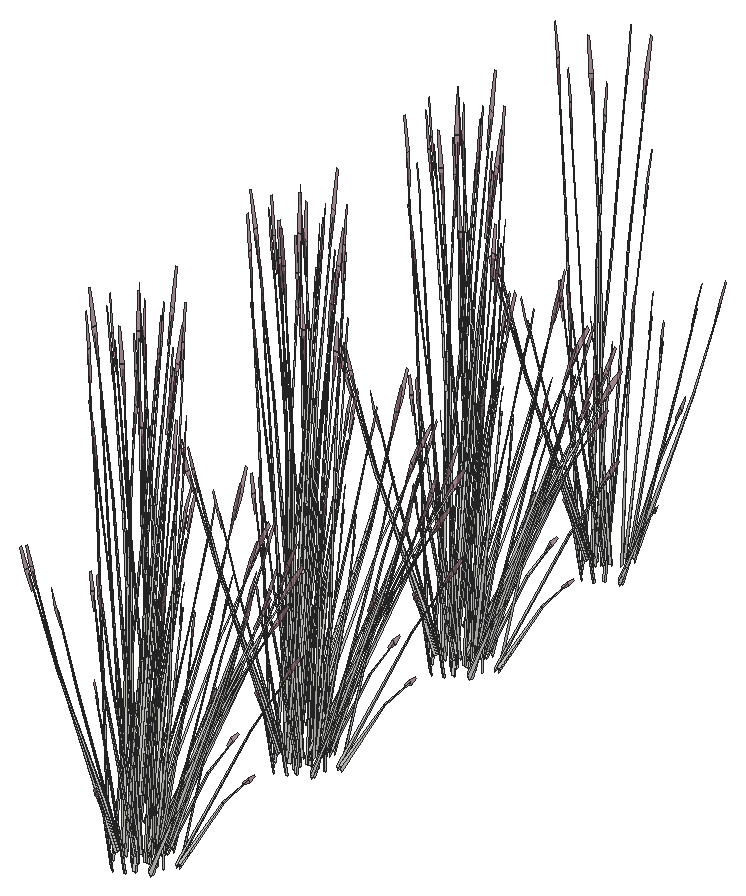
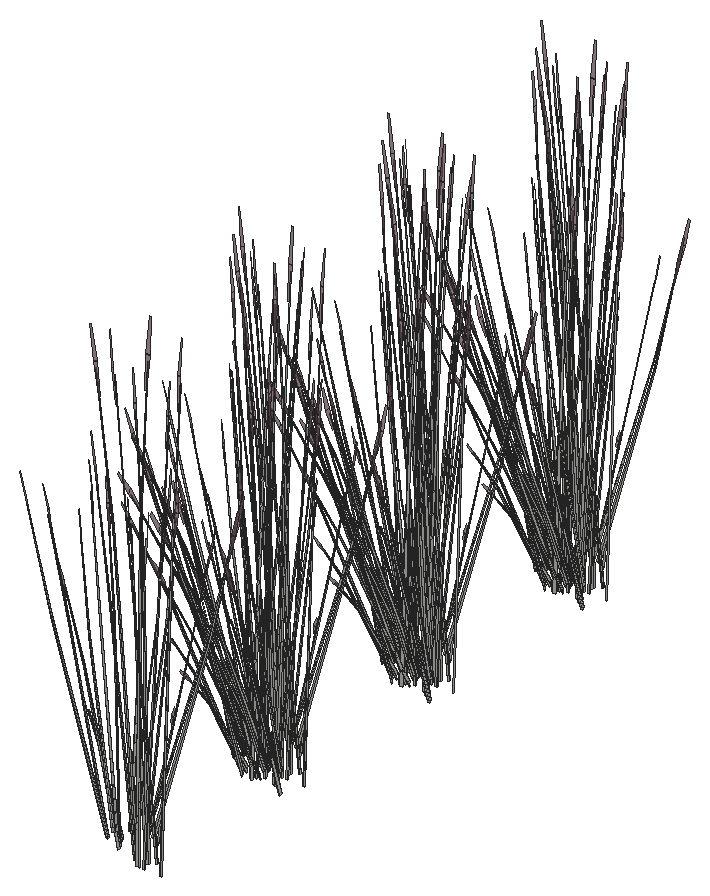
# SketchUp Ruby script. Lengths in inches.
U = 1.inch
M = Sketchup.active_model
def pt(a) = Geom::Point3d.new(a.map { |v| v * U })
def face(e, loops, mat)
  f = e.add_face(loops[0].map { |a| pt(a) })
  loops[1..].each { |l| e.add_face(l.map { |a| pt(a) }).erase! }
  f.material = f.back_material = mat if mat
  f
end
# faces: each face lists its corners as indices into pts; further lists are holes
def faces(e, pts, list, mat = nil) = list.each { |f| face(e, (f[0].is_a?(Array) ? f : [f]).map { |l| l.map { |i| pts[i] } }, mat) }
# xy, xz, yz: faces in a plane at the given z, y or x. An outline is a flat list of corners, or four numbers for a rectangle; further outlines are holes
def ring(l) = l.size == 4 ? [[l[0], l[1]], [l[2], l[1]], [l[2], l[3]], [l[0], l[3]]] : l.each_slice(2).to_a
def flat(e, list, mat, &to3) = list.each { |f| face(e, (f[0].is_a?(Array) ? f : [f]).map { |l| ring(l).map { |u, v| to3.(u, v) } }, mat) }
def xy(e, z, list, mat = nil) = flat(e, list, mat) { |x, y| [x, y, z] }
def xz(e, y, list, mat = nil) = flat(e, list, mat) { |x, z| [x, y, z] }
def yz(e, x, list, mat = nil) = flat(e, list, mat) { |y, z| [x, y, z] }
def lines(e, pts, list) = list.each { |a, b| e.add_line(pt(pts[a]), pt(pts[b])) }
# prism: a flat outline (further loops are holes) pulled along v
def prism(e, loops, v, mat = nil)
  f = face(e, loops, mat); d = Geom::Vector3d.new(v.map { |x| x * U })
  f.pushpull(f.normal.samedirection?(d) ? d.length : -d.length)
end
def box(e, o, s, mat = nil) = prism(e, [[o, [o[0] + s[0], o[1], o[2]], [o[0] + s[0], o[1] + s[1], o[2]], [o[0], o[1] + s[1], o[2]]]], [0, 0, s[2]], mat)
def at(x, y, z, deg = 0) = Geom::Transformation.translation(pt([x, y, z])) * Geom::Transformation.rotation(ORIGIN, Z_AXIS, deg.degrees)
def axes(o, x, y, z) = Geom::Transformation.new([*x, 0, *y, 0, *z, 0, *pt(o).to_a, 1])
def part(name) = M.definitions.add(name)
# library, detail: a bought-in or finely detailed component or shape, given as its bounding box
def library(name, o, s) = part(name).tap { |d| box(d.entities, o, s) }
def detail(e, o, s) = box(e.add_group.entities, o, s)
def put(e, d, t, mat = nil) = e.add_instance(d, t).tap { |i| i.material = mat if mat }
def group(e, t, mat = nil) = e.add_group.tap { |g| g.transformation = t; g.material = mat if mat }.entities
root = M.entities
M.materials.add("LightPink_Translucent").color = [144, 107, 117]
M.materials["LightPink_Translucent"].alpha = 0.75
c1 = part("blade")
p = [[2.15,0.21,22],[0,0.17,0],[0.09,0.45,0],[2.18,0.31,22],[2.29,0.31,22],[0.38,0.45,0],
  [2.48,0.24,33],[2.49,0.24,33],[2.48,0.22,33]]
faces(c1.entities,p,[[0,1,2,3],[4,5,2,3],[6,3,4,7],[8,0,3,6]])
c2 = part("seeds")
p = [[0.3,-0.1,1.38],[-0.01,-0.03,1.59],[-0.01,-0.03,0.03],[0.14,-0.07,-0.07],[0.29,-0.03,3],[0.15,0.01,3.11]]
faces(c2.entities,p,[[0,1,2,3],[1,0,4,5]],"LightPink_Translucent")
c3 = part("blade with seeds")
put(c3.entities,c1,at(0,0,0))
put(c3.entities,c2,axes([2.4,0.25,30.99],[1.5799,-0.05474,1.17369],[-0.12525,1.92788,0.29478],[-0.07173,-0.02425,1.56792]))
put(root,c3,axes([406.6,127.85,258.36],[0.01669,-0.31544,1.54345],[0.75083,0.16661,0.21329],[-0.06506,0.33618,0.72882]))
put(root,c3,axes([407.66,80.2,257.48],[0.7111,0.30552,0.49651],[-0.42504,0.54784,0],[-0.16196,-0.06958,1.57504]))
put(root,c3,axes([406.69,80.9375,258.36],[0.01669,-0.31544,1.54345],[0.75083,0.16661,0.21329],[-0.06506,0.33618,0.72882]))
put(root,c3,axes([405.88,147.62,257.48],[0,0.61104,0.49651],[-0.85008,0,0],[0,-0.13917,1.57504]))
put(root,c3,axes([407.78,103.73,257.48],[0.7111,0.30552,0.49651],[-0.42504,0.54784,0],[-0.16196,-0.06958,1.57504]))
put(root,c3,axes([406.82,104.46,258.36],[0.01669,-0.31544,1.54345],[0.75083,0.16661,0.21329],[-0.06506,0.33618,0.72882]))
put(root,c3,axes([408.58,126.17,257.62],[-0.14658,0.54532,0.1448],[-0.71613,-0.09466,-0.41347],[-0.13033,-0.05599,1.26744]))
put(root,c3,axes([408.67,79.25,257.62],[-0.14658,0.54532,0.1448],[-0.71613,-0.09466,-0.41347],[-0.13033,-0.05599,1.26744]))
put(root,c3,axes([406.16,125.21,257.48],[0,0.61104,0.49651],[-0.85008,0,0],[0,-0.13917,1.57504]))
put(root,c3,axes([406.25,78.3,257.48],[0,0.61104,0.49651],[-0.85008,0,0],[0,-0.13917,1.57504]))
put(root,c3,axes([408.8,102.78,257.62],[-0.14658,0.54532,0.1448],[-0.71613,-0.09466,-0.41347],[-0.13033,-0.05599,1.26744]))
put(root,c3,axes([406.38,101.82,257.48],[0,0.61104,0.49651],[-0.85008,0,0],[0,-0.13917,1.57504]))
put(root,c3,axes([407.04,127.24,260],[0.54391,0.41056,-0.5672],[-0.57458,0.35956,-0.43934],[-0.08276,0.2086,1.08528]))
put(root,c3,axes([407.14,80.33,260],[0.54391,0.41056,-0.5672],[-0.57458,0.35956,-0.43934],[-0.08276,0.2086,1.08528]))
put(root,c3,axes([410.25,125.17,257.84],[-0.02076,-0.57531,1.41272],[0.93937,0.14913,0.59816],[-0.22217,0.31481,1.3335]))
put(root,c3,axes([407.26,103.86,260],[0.54391,0.41056,-0.5672],[-0.57458,0.35956,-0.43934],[-0.08276,0.2086,1.08528]))
put(root,c3,axes([410.34,78.25,257.84],[-0.02076,-0.57531,1.41272],[0.93937,0.14913,0.59816],[-0.22217,0.31481,1.3335]))
put(root,c3,axes([408.76,145.17,259.68],[-0.7469,-0.15318,-0.51099],[0.25601,-0.52518,-0.3958],[-0.06849,-0.21144,0.97773]))
put(root,c3,axes([410.47,101.78,257.84],[-0.02076,-0.57531,1.41272],[0.93937,0.14913,0.59816],[-0.22217,0.31481,1.3335]))
put(root,c3,axes([406.45,127.86,257.82],[0.69024,-0.1082,0.06507],[0.15868,0.43593,-0.86304],[-0.04376,0.22067,0.7736]))
put(root,c3,axes([409.04,122.76,259.68],[-0.7469,-0.15318,-0.51099],[0.25601,-0.52518,-0.3958],[-0.06849,-0.21144,0.97773]))
put(root,c3,axes([406.55,80.95,257.82],[0.69024,-0.1082,0.06507],[0.15868,0.43593,-0.86304],[-0.04376,0.22067,0.7736]))
put(root,c3,axes([409.13,75.85,259.68],[-0.7469,-0.15318,-0.51099],[0.25601,-0.52518,-0.3958],[-0.06849,-0.21144,0.97773]))
put(root,c3,axes([407.66,126.65,258.875],[-0.0186,-0.23452,1.71376],[0.80601,0.15558,0.13857],[-0.04985,0.33422,0.73262]))
put(root,c3,axes([406.67,104.47,257.82],[0.69024,-0.1082,0.06507],[0.15868,0.43593,-0.86304],[-0.04376,0.22067,0.7736]))
put(root,c3,axes([407.76,79.74,258.875],[-0.0186,-0.23452,1.71376],[0.80601,0.15558,0.13857],[-0.04985,0.33422,0.73262]))
put(root,c3,axes([409.26,99.375,259.68],[-0.7469,-0.15318,-0.51099],[0.25601,-0.52518,-0.3958],[-0.06849,-0.21144,0.97773]))
put(root,c3,axes([407.88,103.27,258.875],[-0.0186,-0.23452,1.71376],[0.80601,0.15558,0.13857],[-0.04985,0.33422,0.73262]))
put(root,c3,axes([407.82,147.93,257.72],[-0.36864,0.55059,0.44739],[-0.76598,-0.26498,-0.21531],[0,-0.12692,1.43643]))
put(root,c3,axes([409.03,145.27,259.98],[-0.36264,-0.49684,-0.71045],[0.74649,-0.27689,0.08574],[-0.0848,-0.24006,1.00501]))
put(root,c3,axes([408.1,125.52,257.72],[-0.36864,0.55059,0.44739],[-0.76598,-0.26498,-0.21531],[0,-0.12692,1.43643]))
put(root,c3,axes([409.3125,122.86,259.98],[-0.36264,-0.49684,-0.71045],[0.74649,-0.27689,0.08574],[-0.0848,-0.24006,1.00501]))
put(root,c3,axes([408.1875,78.6,257.72],[-0.36864,0.55059,0.44739],[-0.76598,-0.26498,-0.21531],[0,-0.12692,1.43643]))
put(root,c3,axes([409.41,75.95,259.98],[-0.36264,-0.49684,-0.71045],[0.74649,-0.27689,0.08574],[-0.0848,-0.24006,1.00501]))
put(root,c3,axes([408.3125,102.13,257.72],[-0.36864,0.55059,0.44739],[-0.76598,-0.26498,-0.21531],[0,-0.12692,1.43643]))
put(root,c3,axes([409.53,99.48,259.98],[-0.36264,-0.49684,-0.71045],[0.74649,-0.27689,0.08574],[-0.0848,-0.24006,1.00501]))
put(root,c3,axes([407.83,126.81,257.47],[0.81646,-0.16218,0.17642],[0.20161,0.60355,0.35086],[-0.07282,-0.08794,1.60407]))
put(root,c3,axes([407.92,79.9,257.47],[0.81646,-0.16218,0.17642],[0.20161,0.60355,0.35086],[-0.07282,-0.08794,1.60407]))
put(root,c3,axes([408.05,103.42,257.47],[0.81646,-0.16218,0.17642],[0.20161,0.60355,0.35086],[-0.07282,-0.08794,1.60407]))
put(root,c3,axes([410.26,126.84,257.47],[0.21949,-0.60727,0.17642],[0.8032,0.17185,0.35086],[-0.13875,0.00296,1.60407]))
put(root,c3,axes([409.89,126.04,257.62],[0.56134,0.36712,0.1448],[-0.46823,0.41419,-0.41347],[-0.13033,0.05599,1.26744]))
put(root,c3,axes([410.35,79.93,257.47],[0.21949,-0.60727,0.17642],[0.8032,0.17185,0.35086],[-0.13875,0.00296,1.60407]))
put(root,c3,axes([409.98,79.12,257.62],[0.56134,0.36712,0.1448],[-0.46823,0.41419,-0.41347],[-0.13033,0.05599,1.26744]))
put(root,c3,axes([409.875,125.77,257.72],[0.82508,-0.03772,0.44739],[0.07462,0.62614,-0.21531],[-0.14771,0.06346,1.43643]))
put(root,c3,axes([410.48,103.45,257.47],[0.21949,-0.60727,0.17642],[0.8032,0.17185,0.35086],[-0.13875,0.00296,1.60407]))
put(root,c3,axes([410.11,102.65,257.62],[0.56134,0.36712,0.1448],[-0.46823,0.41419,-0.41347],[-0.13033,0.05599,1.26744]))
put(root,c3,axes([409.1,144.85,259.53],[0.22906,-0.4699,-0.35414],[0.66828,0.13705,0.4572],[-0.06128,-0.18919,0.87481]))
put(root,c3,axes([409.97,78.85,257.72],[0.82508,-0.03772,0.44739],[0.07462,0.62614,-0.21531],[-0.14771,0.06346,1.43643]))
put(root,c3,axes([410.09,102.38,257.72],[0.82508,-0.03772,0.44739],[0.07462,0.62614,-0.21531],[-0.14771,0.06346,1.43643]))
put(root,c3,axes([410.48,127.17,257.48],[0.7111,-0.30552,0.49651],[0.42504,0.54784,0],[-0.16196,0.06958,1.57504]))
put(root,c3,axes([409.38,122.44,259.53],[0.22906,-0.4699,-0.35414],[0.66828,0.13705,0.4572],[-0.06128,-0.18919,0.87481]))
put(root,c3,axes([410.58,80.25,257.48],[0.7111,-0.30552,0.49651],[0.42504,0.54784,0],[-0.16196,0.06958,1.57504]))
put(root,c3,axes([409.47,75.53,259.53],[0.22906,-0.4699,-0.35414],[0.66828,0.13705,0.4572],[-0.06128,-0.18919,0.87481]))
put(root,c3,axes([410.7,103.78,257.48],[0.7111,-0.30552,0.49651],[0.42504,0.54784,0],[-0.16196,0.06958,1.57504]))
put(root,c3,axes([408.32,127.96,259.53],[-0.22906,0.4699,-0.35414],[-0.66828,-0.13705,0.4572],[0.06128,0.18919,0.87481]))
put(root,c3,axes([409.6,99.05,259.53],[0.22906,-0.4699,-0.35414],[0.66828,0.13705,0.4572],[-0.06128,-0.18919,0.87481]))
put(root,c3,axes([408.48,101.59,257.36],[0.33034,0.68327,0.45755],[-0.94388,0.2376,0.17955],[0.01154,-0.12555,1.58856]))
put(root,c3,axes([408.41,81.05,259.53],[-0.22906,0.4699,-0.35414],[-0.66828,-0.13705,0.4572],[0.06128,0.18919,0.87481]))
put(root,c3,axes([408.54,104.58,259.53],[-0.22906,0.4699,-0.35414],[-0.66828,-0.13705,0.4572],[0.06128,0.18919,0.87481]))
put(root,c3,axes([408.29,147.57,257.43],[0.8561,0.29616,0.24065],[-0.41201,0.61537,0.50002],[0,-0.14185,1.60543]))
put(root,c3,axes([408.01,147.16,257.72],[-0.82508,0.03772,0.44739],[-0.07462,-0.62614,-0.21531],[0.14771,-0.06346,1.43643]))
put(root,c3,axes([411.51,125.29,257.47],[-0.59697,-0.44509,0.17642],[0.60159,-0.4317,0.35086],[-0.06593,0.0909,1.60407]))
put(root,c3,axes([407.63,146.09,257.47],[-0.21949,0.60727,0.17642],[-0.8032,-0.17185,0.35086],[0.13875,-0.00296,1.60407]))
put(root,c3,axes([411.61,78.38,257.47],[-0.59697,-0.44509,0.17642],[0.60159,-0.4317,0.35086],[-0.06593,0.0909,1.60407]))
put(root,c3,axes([408.57,125.16,257.43],[0.8561,0.29616,0.24065],[-0.41201,0.61537,0.50002],[0,-0.14185,1.60543]))
put(root,c3,axes([408.29,124.75,257.72],[-0.82508,0.03772,0.44739],[-0.07462,-0.62614,-0.21531],[0.14771,-0.06346,1.43643]))
put(root,c3,axes([411.73,101.91,257.47],[-0.59697,-0.44509,0.17642],[0.60159,-0.4317,0.35086],[-0.06593,0.0909,1.60407]))
put(root,c3,axes([408.66,78.25,257.43],[0.8561,0.29616,0.24065],[-0.41201,0.61537,0.50002],[0,-0.14185,1.60543]))
put(root,c3,axes([408.38,77.84,257.72],[-0.82508,0.03772,0.44739],[-0.07462,-0.62614,-0.21531],[0.14771,-0.06346,1.43643]))
put(root,c3,axes([408.79,101.78,257.43],[0.8561,0.29616,0.24065],[-0.41201,0.61537,0.50002],[0,-0.14185,1.60543]))
put(root,c3,axes([407.91,123.68,257.47],[-0.21949,0.60727,0.17642],[-0.8032,-0.17185,0.35086],[0.13875,-0.00296,1.60407]))
put(root,c3,axes([408.51,101.36,257.72],[-0.82508,0.03772,0.44739],[-0.07462,-0.62614,-0.21531],[0.14771,-0.06346,1.43643]))
put(root,c3,axes([408,76.76,257.47],[-0.21949,0.60727,0.17642],[-0.8032,-0.17185,0.35086],[0.13875,-0.00296,1.60407]))
put(root,c3,axes([408.125,100.29,257.47],[-0.21949,0.60727,0.17642],[-0.8032,-0.17185,0.35086],[0.13875,-0.00296,1.60407]))
put(root,c3,axes([408.39,127.54,259.98],[0.36264,0.49684,-0.71045],[-0.74649,0.27689,0.08574],[0.0848,0.24006,1.00501]))
put(root,c3,axes([409.22,143.86,257.77],[0.09747,0.35631,1.1486],[-0.54071,-0.19735,0.84392],[0.05818,-0.18244,0.25299]))
put(root,c3,axes([408.48,80.63,259.98],[0.36264,0.49684,-0.71045],[-0.74649,0.27689,0.08574],[0.0848,0.24006,1.00501]))
put(root,c3,axes([410.34,123.71,257.47],[-0.81646,0.16218,0.17642],[-0.20161,-0.60355,0.35086],[0.07282,0.08794,1.60407]))
put(root,c3,axes([408.6,104.15,259.98],[0.36264,0.49684,-0.71045],[-0.74649,0.27689,0.08574],[0.0848,0.24006,1.00501]))
put(root,c3,axes([410.43,76.8,257.47],[-0.81646,0.16218,0.17642],[-0.20161,-0.60355,0.35086],[0.07282,0.08794,1.60407]))
put(root,c3,axes([409.5,121.45,257.77],[0.09747,0.35631,1.1486],[-0.54071,-0.19735,0.84392],[0.05818,-0.18244,0.25299]))
put(root,c3,axes([410.55,100.32,257.47],[-0.81646,0.16218,0.17642],[-0.20161,-0.60355,0.35086],[0.07282,0.08794,1.60407]))
put(root,c3,axes([409.6,74.53,257.77],[0.09747,0.35631,1.1486],[-0.54071,-0.19735,0.84392],[0.05818,-0.18244,0.25299]))
put(root,c3,axes([410.07,125,257.72],[0.36864,-0.55059,0.44739],[0.76598,0.26498,-0.21531],[0,0.12692,1.43643]))
put(root,c3,axes([409.72,98.0625,257.77],[0.09747,0.35631,1.1486],[-0.54071,-0.19735,0.84392],[0.05818,-0.18244,0.25299]))
put(root,c3,axes([410.16,78.09,257.72],[0.36864,-0.55059,0.44739],[0.76598,0.26498,-0.21531],[0,0.12692,1.43643]))
put(root,c3,axes([409.22,101.2,257.36],[-0.62999,0.55453,0.45755],[-0.74845,-0.4895,0.17955],[0.15188,-0.05534,1.58856]))
put(root,c3,axes([408.66,127.64,259.68],[0.7469,0.15318,-0.51099],[-0.25601,0.52518,-0.3958],[0.06849,0.21144,0.97773]))
put(root,c3,axes([410.29,101.62,257.72],[0.36864,-0.55059,0.44739],[0.76598,0.26498,-0.21531],[0,0.12692,1.43643]))
put(root,c3,axes([408.75,80.73,259.68],[0.7469,0.15318,-0.51099],[-0.25601,0.52518,-0.3958],[0.06849,0.21144,0.97773]))
put(root,c3,axes([409.82,124.87,257.38],[-0.96033,-0.12874,0.49198],[0.19544,-0.7271,0.19306],[0.14034,0.07021,1.70813]))
put(root,c3,axes([409.91,77.96,257.38],[-0.96033,-0.12874,0.49198],[0.19544,-0.7271,0.19306],[0.14034,0.07021,1.70813]))
put(root,c3,axes([408.875,104.25,259.68],[0.7469,0.15318,-0.51099],[-0.25601,0.52518,-0.3958],[0.06849,0.21144,0.97773]))
put(root,c3,axes([410.375,145.57,259.68],[-0.54391,-0.41056,-0.51099],[0.57458,-0.35956,-0.3958],[0.08276,-0.2086,0.97773]))
put(root,c3,axes([410.04,101.48,257.38],[-0.96033,-0.12874,0.49198],[0.19544,-0.7271,0.19306],[0.14034,0.07021,1.70813]))
put(root,c3,axes([409.28,124.49,257.72],[-0.45644,-0.51287,0.44739],[0.69137,-0.36116,-0.21531],[0.14771,0.06346,1.43643]))
put(root,c3,axes([410.39,125.13,257.62],[0.70791,-0.1782,0.1448],[0.24791,0.50885,-0.41347],[0,0.11199,1.26744]))
put(root,c3,axes([410.65,123.16,259.68],[-0.54391,-0.41056,-0.51099],[0.57458,-0.35956,-0.3958],[0.08276,-0.2086,0.97773]))
put(root,c3,axes([409.37,77.58,257.72],[-0.45644,-0.51287,0.44739],[0.69137,-0.36116,-0.21531],[0.14771,0.06346,1.43643]))
put(root,c3,axes([410.48,78.22,257.62],[0.70791,-0.1782,0.1448],[0.24791,0.50885,-0.41347],[0,0.11199,1.26744]))
put(root,c3,axes([410.75,76.25,259.68],[-0.54391,-0.41056,-0.51099],[0.57458,-0.35956,-0.3958],[0.08276,-0.2086,0.97773]))
put(root,c3,axes([409.5,101.11,257.72],[-0.45644,-0.51287,0.44739],[0.69137,-0.36116,-0.21531],[0.14771,0.06346,1.43643]))
put(root,c3,axes([410.61,101.74,257.62],[0.70791,-0.1782,0.1448],[0.24791,0.50885,-0.41347],[0,0.11199,1.26744]))
put(root,c3,axes([410.87,99.77,259.68],[-0.54391,-0.41056,-0.51099],[0.57458,-0.35956,-0.3958],[0.08276,-0.2086,0.97773]))
put(root,c3,axes([410.02,144.84,257.59],[-0.21597,0.12368,1.43002],[-0.64681,-0.21647,-0.30754],[0.1199,-0.26922,0.61141]))
put(root,c3,axes([410.3,122.43,257.59],[-0.21597,0.12368,1.43002],[-0.64681,-0.21647,-0.30754],[0.1199,-0.26922,0.61141]))
put(root,c3,axes([409.31,146.76,257.62],[0.14658,-0.54532,0.1448],[0.71613,0.09466,-0.41347],[0.13033,0.05599,1.26744]))
put(root,c3,axes([410.39,75.52,257.59],[-0.21597,0.12368,1.43002],[-0.64681,-0.21647,-0.30754],[0.1199,-0.26922,0.61141]))
put(root,c3,axes([412,125.31,257.48],[0,-0.61104,0.49651],[0.85008,0,0],[0,0.13917,1.57504]))
put(root,c3,axes([410.52,99.05,257.59],[-0.21597,0.12368,1.43002],[-0.64681,-0.21647,-0.30754],[0.1199,-0.26922,0.61141]))
put(root,c3,axes([412.1,78.4,257.48],[0,-0.61104,0.49651],[0.85008,0,0],[0,0.13917,1.57504]))
put(root,c3,axes([409.08,126.56,258.875],[-0.17368,-0.19618,1.71376],[0.80256,-0.16516,0.13857],[0.18139,0.30799,0.73262]))
put(root,c3,axes([409.58,124.35,257.62],[0.14658,-0.54532,0.1448],[0.71613,0.09466,-0.41347],[0.13033,0.05599,1.26744]))
put(root,c3,axes([410.32,145.8125,257.48],[-0.7111,-0.30552,0.49651],[0.42504,-0.54784,0],[0.16196,0.06958,1.57504]))
put(root,c3,axes([410.54,145.76,259.98],[0.01977,-0.56521,-0.71045],[0.83252,0.03796,0.08574],[0.08786,-0.23945,1.00501]))
put(root,c3,axes([409.17,79.64,258.875],[-0.17368,-0.19618,1.71376],[0.80256,-0.16516,0.13857],[0.18139,0.30799,0.73262]))
put(root,c3,axes([409.68,77.4375,257.62],[0.14658,-0.54532,0.1448],[0.71613,0.09466,-0.41347],[0.13033,0.05599,1.26744]))
put(root,c3,axes([412.22,101.92,257.48],[0,-0.61104,0.49651],[0.85008,0,0],[0,0.13917,1.57504]))
put(root,c3,axes([409.3,103.17,258.875],[-0.17368,-0.19618,1.71376],[0.80256,-0.16516,0.13857],[0.18139,0.30799,0.73262]))
put(root,c3,axes([409.8,100.96,257.62],[0.14658,-0.54532,0.1448],[0.71613,0.09466,-0.41347],[0.13033,0.05599,1.26744]))
put(root,c3,axes([410.6,123.4,257.48],[-0.7111,-0.30552,0.49651],[0.42504,-0.54784,0],[0.16196,0.06958,1.57504]))
put(root,c3,axes([410.82,123.35,259.98],[0.01977,-0.56521,-0.71045],[0.83252,0.03796,0.08574],[0.08786,-0.23945,1.00501]))
put(root,c3,axes([410.7,76.49,257.48],[-0.7111,-0.30552,0.49651],[0.42504,-0.54784,0],[0.16196,0.06958,1.57504]))
put(root,c3,axes([410.92,76.44,259.98],[0.01977,-0.56521,-0.71045],[0.83252,0.03796,0.08574],[0.08786,-0.23945,1.00501]))
put(root,c3,axes([410.82,100.01,257.48],[-0.7111,-0.30552,0.49651],[0.42504,-0.54784,0],[0.16196,0.06958,1.57504]))
put(root,c3,axes([411.04,99.96,259.98],[0.01977,-0.56521,-0.71045],[0.83252,0.03796,0.08574],[0.08786,-0.23945,1.00501]))
put(root,c3,axes([410.89,145.42,259.53],[0.5141,-0.32171,-0.35414],[0.48666,0.36734,0.4572],[0.07405,-0.18664,0.87481]))
put(root,c3,axes([411.17,123.01,259.53],[0.5141,-0.32171,-0.35414],[0.48666,0.36734,0.4572],[0.07405,-0.18664,0.87481]))
put(root,c3,axes([411.26,76.1,259.53],[0.5141,-0.32171,-0.35414],[0.48666,0.36734,0.4572],[0.07405,-0.18664,0.87481]))
put(root,c3,axes([411.29,127.14,257.77],[-0.4278,-0.1757,1.1486],[0.5524,-0.17852,0.84392],[0.14899,0.15122,0.25299]))
put(root,c3,axes([409.77,126.96,257.59],[0.01341,-0.20255,1.43002],[0.64074,-0.22625,-0.30754],[0.1978,0.24243,0.61141]))
put(root,c3,axes([411.38,99.62,259.53],[0.5141,-0.32171,-0.35414],[0.48666,0.36734,0.4572],[0.07405,-0.18664,0.87481]))
put(root,c3,axes([411.38,80.23,257.77],[-0.4278,-0.1757,1.1486],[0.5524,-0.17852,0.84392],[0.14899,0.15122,0.25299]))
put(root,c3,axes([409.86,80.04,257.59],[0.01341,-0.20255,1.43002],[0.64074,-0.22625,-0.30754],[0.1978,0.24243,0.61141]))
put(root,c3,axes([411.51,103.76,257.77],[-0.4278,-0.1757,1.1486],[0.5524,-0.17852,0.84392],[0.14899,0.15122,0.25299]))
put(root,c3,axes([409.98,103.57,257.59],[0.01341,-0.20255,1.43002],[0.64074,-0.22625,-0.30754],[0.1978,0.24243,0.61141]))
put(root,c3,axes([409.61,145.47,258.875],[-0.14147,0.21002,1.71376],[-0.59349,-0.43464,0.13857],[0.26773,-0.27089,0.73262]))
put(root,c3,axes([411.36,127.94,257.67],[-0.48723,-0.01916,1.0506],[0.32177,-0.40701,0.58006],[0.19248,0.1446,0.8241]))
put(root,c3,axes([411.45,81.03,257.67],[-0.48723,-0.01916,1.0506],[0.32177,-0.40701,0.58006],[0.19248,0.1446,0.8241]))
put(root,c3,axes([409.89,123.0625,258.875],[-0.14147,0.21002,1.71376],[-0.59349,-0.43464,0.13857],[0.26773,-0.27089,0.73262]))
put(root,c3,axes([411.58,104.56,257.67],[-0.48723,-0.01916,1.0506],[0.32177,-0.40701,0.58006],[0.19248,0.1446,0.8241]))
put(root,c3,axes([409.98,76.15,258.875],[-0.14147,0.21002,1.71376],[-0.59349,-0.43464,0.13857],[0.26773,-0.27089,0.73262]))
put(root,c3,axes([410.1,99.67,258.875],[-0.14147,0.21002,1.71376],[-0.59349,-0.43464,0.13857],[0.26773,-0.27089,0.73262]))
put(root,c3,axes([410.32,127.39,259.68],[0.74975,-0.14525,-0.51099],[0.13115,0.55007,-0.3958],[0.20138,0.15763,0.97773]))
put(root,c3,axes([410.42,80.47,259.68],[0.74975,-0.14525,-0.51099],[0.13115,0.55007,-0.3958],[0.20138,0.15763,0.97773]))
put(root,c3,axes([411.51,146.52,259.68],[-0.19519,-0.55794,-0.51099],[0.73919,-0.0976,-0.3958],[0.21183,-0.14986,0.97773]))
put(root,c3,axes([410.54,104,259.68],[0.74975,-0.14525,-0.51099],[0.13115,0.55007,-0.3958],[0.20138,0.15763,0.97773]))
put(root,c3,axes([411.78,124.11,259.68],[-0.19519,-0.55794,-0.51099],[0.73919,-0.0976,-0.3958],[0.21183,-0.14986,0.97773]))
put(root,c3,axes([411.88,77.19,259.68],[-0.19519,-0.55794,-0.51099],[0.73919,-0.0976,-0.3958],[0.21183,-0.14986,0.97773]))
put(root,c3,axes([413.08,126.98,258.93],[-0.14542,-0.51365,-0.03492],[0.68734,-0.11809,-0.15832],[0.14353,0.03256,0.52218]))
put(root,c3,axes([413.18,80.07,258.93],[-0.14542,-0.51365,-0.03492],[0.68734,-0.11809,-0.15832],[0.14353,0.03256,0.52218]))
put(root,c3,axes([412,100.72,259.68],[-0.19519,-0.55794,-0.51099],[0.73919,-0.0976,-0.3958],[0.21183,-0.14986,0.97773]))
put(root,c3,axes([412.41,145.41,257.77],[-0.25308,0.31105,1.1486],[-0.21753,-0.4179,0.84392],[0.20902,-0.10472,0.25299]))
put(root,c3,axes([413.3,103.6,258.93],[-0.14542,-0.51365,-0.03492],[0.68734,-0.11809,-0.15832],[0.14353,0.03256,0.52218]))
put(root,c3,axes([412.69,123,257.77],[-0.25308,0.31105,1.1486],[-0.21753,-0.4179,0.84392],[0.20902,-0.10472,0.25299]))
put(root,c3,axes([412.78,76.08,257.77],[-0.25308,0.31105,1.1486],[-0.21753,-0.4179,0.84392],[0.20902,-0.10472,0.25299]))
put(root,c3,axes([412.91,99.61,257.77],[-0.25308,0.31105,1.1486],[-0.21753,-0.4179,0.84392],[0.20902,-0.10472,0.25299]))
put(root,c3,axes([412.05,146.57,259.53],[0.66138,-0.08733,-0.35414],[0.17464,0.49921,0.4572],[0.18953,-0.13408,0.87481]))
put(root,c3,axes([411.53,146.74,259.98],[0.39688,-0.48213,-0.71045],[0.69548,0.34264,0.08574],[0.23697,-0.17468,1.00501]))
put(root,c3,axes([410.24,125.95,258.875],[-0.28223,-0.10528,1.71376],[0.58406,-0.44165,0.13857],[0.36402,0.19924,0.73262]))
put(root,c3,axes([410.34,79.03,258.875],[-0.28223,-0.10528,1.71376],[0.58406,-0.44165,0.13857],[0.36402,0.19924,0.73262]))
put(root,c3,axes([412.33,124.16,259.53],[0.66138,-0.08733,-0.35414],[0.17464,0.49921,0.4572],[0.18953,-0.13408,0.87481]))
put(root,c3,axes([410.46,102.56,258.875],[-0.28223,-0.10528,1.71376],[0.58406,-0.44165,0.13857],[0.36402,0.19924,0.73262]))
put(root,c3,axes([411.8,124.33,259.98],[0.39688,-0.48213,-0.71045],[0.69548,0.34264,0.08574],[0.23697,-0.17468,1.00501]))
put(root,c3,axes([412.42,77.25,259.53],[0.66138,-0.08733,-0.35414],[0.17464,0.49921,0.4572],[0.18953,-0.13408,0.87481]))
put(root,c3,axes([411.8,126.93,259.53],[0.43232,0.38257,-0.35414],[-0.49364,0.36215,0.4572],[0.25081,0.0551,0.87481]))
put(root,c3,axes([411.9,77.42,259.98],[0.39688,-0.48213,-0.71045],[0.69548,0.34264,0.08574],[0.23697,-0.17468,1.00501]))
put(root,c3,axes([411.89,80.01,259.53],[0.43232,0.38257,-0.35414],[-0.49364,0.36215,0.4572],[0.25081,0.0551,0.87481]))
put(root,c3,axes([412.55,100.78,259.53],[0.66138,-0.08733,-0.35414],[0.17464,0.49921,0.4572],[0.18953,-0.13408,0.87481]))
put(root,c3,axes([412.02,100.94,259.98],[0.39688,-0.48213,-0.71045],[0.69548,0.34264,0.08574],[0.23697,-0.17468,1.00501]))
put(root,c3,axes([412.02,103.54,259.53],[0.43232,0.38257,-0.35414],[-0.49364,0.36215,0.4572],[0.25081,0.0551,0.87481]))
put(root,c3,axes([411.85,147.75,259.68],[0.20584,-0.55581,-0.51099],[0.70573,0.19051,-0.3958],[0.28414,-0.05097,0.97773]))
put(root,c3,axes([412.1,146.3,257.59],[-0.27143,-0.0181,1.43002],[-0.27808,-0.48551,-0.30754],[0.33346,-0.13735,0.61141]))
put(root,c3,axes([412.13,125.34,259.68],[0.20584,-0.55581,-0.51099],[0.70573,0.19051,-0.3958],[0.28414,-0.05097,0.97773]))
put(root,c3,axes([413.9,125.7,257.77],[-0.46945,0.10088,1.1486],[0.22097,-0.4169,0.84392],[0.24904,0.02853,0.25299]))
put(root,c3,axes([412.22,78.43,259.68],[0.20584,-0.55581,-0.51099],[0.70573,0.19051,-0.3958],[0.28414,-0.05097,0.97773]))
put(root,c3,axes([413.99,78.79,257.77],[-0.46945,0.10088,1.1486],[0.22097,-0.4169,0.84392],[0.24904,0.02853,0.25299]))
put(root,c3,axes([412.35,101.96,259.68],[0.20584,-0.55581,-0.51099],[0.70573,0.19051,-0.3958],[0.28414,-0.05097,0.97773]))
put(root,c3,axes([412.38,123.89,257.59],[-0.27143,-0.0181,1.43002],[-0.27808,-0.48551,-0.30754],[0.33346,-0.13735,0.61141]))
put(root,c3,axes([414.12,102.3125,257.77],[-0.46945,0.10088,1.1486],[0.22097,-0.4169,0.84392],[0.24904,0.02853,0.25299]))
put(root,c3,axes([412.56,125.6,259.53],[0.63144,0.17046,-0.35414],[-0.18417,0.49731,0.4572],[0.25423,-0.0456,0.87481]))
put(root,c3,axes([412.47,76.97,257.59],[-0.27143,-0.0181,1.43002],[-0.27808,-0.48551,-0.30754],[0.33346,-0.13735,0.61141]))
put(root,c3,axes([412.65,78.69,259.53],[0.63144,0.17046,-0.35414],[-0.18417,0.49731,0.4572],[0.25423,-0.0456,0.87481]))
put(root,c3,axes([412.6,100.5,257.59],[-0.27143,-0.0181,1.43002],[-0.27808,-0.48551,-0.30754],[0.33346,-0.13735,0.61141]))
put(root,c3,axes([411.34,126.67,259.98],[0.75952,0.01471,-0.71045],[-0.05101,0.61953,0.08574],[0.32177,0.06538,1.00501]))
put(root,c3,axes([412.78,102.21,259.53],[0.63144,0.17046,-0.35414],[-0.18417,0.49731,0.4572],[0.25423,-0.0456,0.87481]))
put(root,c3,axes([411.43,79.76,259.98],[0.75952,0.01471,-0.71045],[-0.05101,0.61953,0.08574],[0.32177,0.06538,1.00501]))
put(root,c3,axes([411.56,103.28,259.98],[0.75952,0.01471,-0.71045],[-0.05101,0.61953,0.08574],[0.32177,0.06538,1.00501]))
put(root,c3,axes([410.84,124.98,258.875],[-0.31515,0.01384,1.71376],[0.20907,-0.5998,0.13857],[0.44912,0.0371,0.73262]))
put(root,c3,axes([411.71,147.96,259.98],[0.66765,-0.26986,-0.71045],[0.37208,0.55551,0.08574],[0.32259,-0.0631,1.00501]))
put(root,c3,axes([410.93,78.07,258.875],[-0.31515,0.01384,1.71376],[0.20907,-0.5998,0.13857],[0.44912,0.0371,0.73262]))
put(root,c3,axes([411.06,101.6,258.875],[-0.31515,0.01384,1.71376],[0.20907,-0.5998,0.13857],[0.44912,0.0371,0.73262]))
put(root,c3,axes([411.99,125.55,259.98],[0.66765,-0.26986,-0.71045],[0.37208,0.55551,0.08574],[0.32259,-0.0631,1.00501]))
put(root,c3,axes([412.09,78.63,259.98],[0.66765,-0.26986,-0.71045],[0.37208,0.55551,0.08574],[0.32259,-0.0631,1.00501]))
put(root,c3,axes([412.21,102.16,259.98],[0.66765,-0.26986,-0.71045],[0.37208,0.55551,0.08574],[0.32259,-0.0631,1.00501]))
put(root,c3,axes([413.02,126.37,257.59],[-0.18299,-0.15028,1.43002],[0.23809,-0.49714,-0.30754],[0.37023,0.06735,0.61141]))
put(root,c3,axes([413.11,79.46,257.59],[-0.18299,-0.15028,1.43002],[0.23809,-0.49714,-0.30754],[0.37023,0.06735,0.61141]))
put(root,c3,axes([413.24,102.98,257.59],[-0.18299,-0.15028,1.43002],[0.23809,-0.49714,-0.30754],[0.37023,0.06735,0.61141]))
